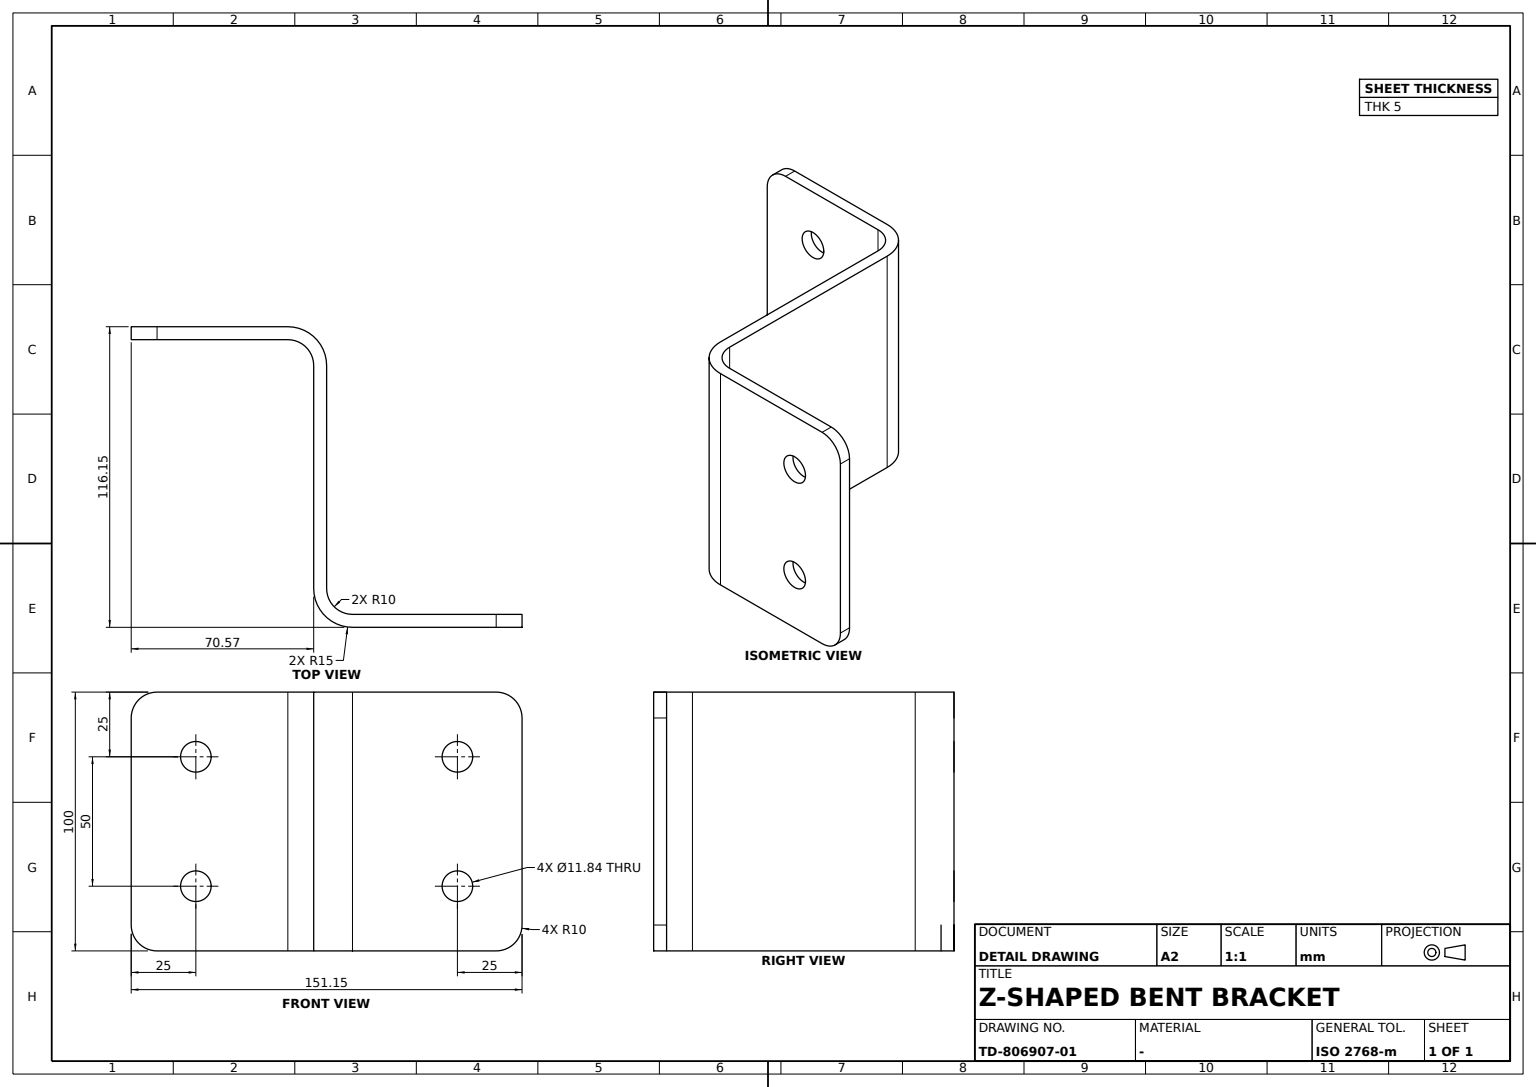
ISO-10303-21;
HEADER;
FILE_DESCRIPTION((''),'2;1');
FILE_NAME('','',(''),(''),'','','');
FILE_SCHEMA(('AUTOMOTIVE_DESIGN'));
ENDSEC;
DATA;
#1=APPLICATION_CONTEXT('');
#2=PRODUCT_CONTEXT('',#1,'mechanical');
#3=PRODUCT('','','',(#2));
#4=PRODUCT_DEFINITION_FORMATION('','',#3);
#5=PRODUCT_DEFINITION_CONTEXT('',#1,'design');
#6=PRODUCT_DEFINITION('','',#4,#5);
#7=PRODUCT_DEFINITION_SHAPE('','',#6);
#8=(LENGTH_UNIT()NAMED_UNIT(*)SI_UNIT(.MILLI.,.METRE.));
#9=(NAMED_UNIT(*)PLANE_ANGLE_UNIT()SI_UNIT($,.RADIAN.));
#10=(NAMED_UNIT(*)SI_UNIT($,.STERADIAN.)SOLID_ANGLE_UNIT());
#11=UNCERTAINTY_MEASURE_WITH_UNIT(LENGTH_MEASURE(0.005),#8,'distance_accuracy_value','');
#12=(GEOMETRIC_REPRESENTATION_CONTEXT(3)GLOBAL_UNCERTAINTY_ASSIGNED_CONTEXT((#11))GLOBAL_UNIT_ASSIGNED_CONTEXT((#8,#9,#10))REPRESENTATION_CONTEXT('',''));
#13=CARTESIAN_POINT('',(-175.5732,49.4268,40.));
#14=VERTEX_POINT('',#13);
#15=CARTESIAN_POINT('',(-175.5732,44.4268,40.));
#16=VERTEX_POINT('',#15);
#17=DIRECTION('',(0.,-1.,0.));
#18=VECTOR('',#17,1000.);
#19=LINE('',#13,#18);
#20=EDGE_CURVE('',#14,#16,#19,.T.);
#21=ORIENTED_EDGE('',*,*,#20,.F.);
#22=CARTESIAN_POINT('',(-175.5732,49.4268,-40.));
#23=VERTEX_POINT('',#22);
#24=CARTESIAN_POINT('',(-175.5732,49.4268,0.));
#25=DIRECTION('',(0.,0.,-1.));
#26=VECTOR('',#25,1000.);
#27=LINE('',#24,#26);
#28=EDGE_CURVE('',#14,#23,#27,.T.);
#29=ORIENTED_EDGE('',*,*,#28,.T.);
#30=CARTESIAN_POINT('',(-175.5732,44.4268,-40.));
#31=VERTEX_POINT('',#30);
#32=LINE('',#22,#18);
#33=EDGE_CURVE('',#23,#31,#32,.T.);
#34=ORIENTED_EDGE('',*,*,#33,.T.);
#35=CARTESIAN_POINT('',(-175.5732,44.4268,0.));
#36=LINE('',#35,#26);
#37=EDGE_CURVE('',#16,#31,#36,.T.);
#38=ORIENTED_EDGE('',*,*,#37,.F.);
#39=EDGE_LOOP('',(#21,#29,#34,#38));
#40=FACE_BOUND('',#39,.T.);
#41=CARTESIAN_POINT('',(-175.5732,49.4268,50.));
#42=DIRECTION('',(-1.,0.,0.));
#43=AXIS2_PLACEMENT_3D('',#41,#42,#25);
#44=PLANE('',#43);
#45=ADVANCED_FACE('',(#40),#44,.T.);
#46=CARTESIAN_POINT('',(-90.,-66.719599,50.));
#47=VERTEX_POINT('',#46);
#48=CARTESIAN_POINT('',(-90.,-66.719599,-50.));
#49=VERTEX_POINT('',#48);
#50=LINE('',#46,#26);
#51=EDGE_CURVE('',#47,#49,#50,.T.);
#52=ORIENTED_EDGE('',*,*,#51,.T.);
#53=CARTESIAN_POINT('',(-34.426804,-66.719599,-50.));
#54=VERTEX_POINT('',#53);
#55=CARTESIAN_POINT('',(-100.,-66.719599,-50.));
#56=DIRECTION('',(1.,0.,0.));
#57=VECTOR('',#56,1000.);
#58=LINE('',#55,#57);
#59=EDGE_CURVE('',#54,#49,#58,.F.);
#60=ORIENTED_EDGE('',*,*,#59,.F.);
#61=CARTESIAN_POINT('',(-24.4268,-66.719599,-40.));
#62=VERTEX_POINT('',#61);
#63=CARTESIAN_POINT('',(-34.4268,-66.719599,-40.));
#64=AXIS2_PLACEMENT_3D('',#63,#17,#56);
#65=CIRCLE('',#64,10.);
#66=EDGE_CURVE('',#62,#54,#65,.F.);
#67=ORIENTED_EDGE('',*,*,#66,.F.);
#68=CARTESIAN_POINT('',(-24.4268,-66.719599,40.));
#69=VERTEX_POINT('',#68);
#70=CARTESIAN_POINT('',(-24.4268,-66.719599,0.));
#71=DIRECTION('',(0.,0.,1.));
#72=VECTOR('',#71,1000.);
#73=LINE('',#70,#72);
#74=EDGE_CURVE('',#62,#69,#73,.T.);
#75=ORIENTED_EDGE('',*,*,#74,.T.);
#76=CARTESIAN_POINT('',(-34.4268,-66.719599,50.));
#77=VERTEX_POINT('',#76);
#78=CARTESIAN_POINT('',(-34.4268,-66.719599,40.));
#79=AXIS2_PLACEMENT_3D('',#78,#17,#56);
#80=CIRCLE('',#79,10.);
#81=EDGE_CURVE('',#77,#69,#80,.F.);
#82=ORIENTED_EDGE('',*,*,#81,.F.);
#83=CARTESIAN_POINT('',(0.,-66.719599,50.));
#84=LINE('',#83,#57);
#85=EDGE_CURVE('',#47,#77,#84,.T.);
#86=ORIENTED_EDGE('',*,*,#85,.F.);
#87=EDGE_LOOP('',(#52,#60,#67,#75,#82,#86));
#88=FACE_BOUND('',#87,.T.);
#89=CARTESIAN_POINT('',(-43.5093,-66.719599,25.));
#90=VERTEX_POINT('',#89);
#91=CARTESIAN_POINT('',(-49.4268,-66.719599,25.));
#92=AXIS2_PLACEMENT_3D('',#91,#17,#56);
#93=CIRCLE('',#92,5.9175);
#94=EDGE_CURVE('',#90,#90,#93,.T.);
#95=ORIENTED_EDGE('',*,*,#94,.F.);
#96=EDGE_LOOP('',(#95));
#97=FACE_BOUND('',#96,.T.);
#98=CARTESIAN_POINT('',(-43.5093,-66.719599,-25.));
#99=VERTEX_POINT('',#98);
#100=CARTESIAN_POINT('',(-49.4268,-66.719599,-25.));
#101=AXIS2_PLACEMENT_3D('',#100,#17,#56);
#102=CIRCLE('',#101,5.9175);
#103=EDGE_CURVE('',#99,#99,#102,.T.);
#104=ORIENTED_EDGE('',*,*,#103,.F.);
#105=EDGE_LOOP('',(#104));
#106=FACE_BOUND('',#105,.T.);
#107=CARTESIAN_POINT('',(-149.4268,-66.719599,0.));
#108=AXIS2_PLACEMENT_3D('',#107,#17,#56);
#109=PLANE('',#108);
#110=ADVANCED_FACE('',(#88,#97,#106),#109,.T.);
#111=CARTESIAN_POINT('',(-24.4268,-61.719599,-40.));
#112=VERTEX_POINT('',#111);
#113=LINE('',#111,#18);
#114=EDGE_CURVE('',#112,#62,#113,.T.);
#115=ORIENTED_EDGE('',*,*,#114,.F.);
#116=CARTESIAN_POINT('',(-24.4268,-61.719599,40.));
#117=VERTEX_POINT('',#116);
#118=CARTESIAN_POINT('',(-24.4268,-61.719599,0.));
#119=LINE('',#118,#72);
#120=EDGE_CURVE('',#112,#117,#119,.T.);
#121=ORIENTED_EDGE('',*,*,#120,.T.);
#122=LINE('',#116,#18);
#123=EDGE_CURVE('',#117,#69,#122,.T.);
#124=ORIENTED_EDGE('',*,*,#123,.T.);
#125=ORIENTED_EDGE('',*,*,#74,.F.);
#126=EDGE_LOOP('',(#115,#121,#124,#125));
#127=FACE_BOUND('',#126,.T.);
#128=CARTESIAN_POINT('',(-24.4268,-61.719599,-50.));
#129=AXIS2_PLACEMENT_3D('',#128,#56,#71);
#130=PLANE('',#129);
#131=ADVANCED_FACE('',(#127),#130,.T.);
#132=CARTESIAN_POINT('',(-105.,34.4268,50.));
#133=VERTEX_POINT('',#132);
#134=CARTESIAN_POINT('',(-105.,34.4268,-50.));
#135=VERTEX_POINT('',#134);
#136=LINE('',#132,#26);
#137=EDGE_CURVE('',#133,#135,#136,.T.);
#138=ORIENTED_EDGE('',*,*,#137,.T.);
#139=CARTESIAN_POINT('',(-105.,-51.719599,-50.));
#140=VERTEX_POINT('',#139);
#141=LINE('',#134,#18);
#142=EDGE_CURVE('',#140,#135,#141,.F.);
#143=ORIENTED_EDGE('',*,*,#142,.F.);
#144=CARTESIAN_POINT('',(-105.,-51.719599,50.));
#145=VERTEX_POINT('',#144);
#146=LINE('',#144,#26);
#147=EDGE_CURVE('',#145,#140,#146,.T.);
#148=ORIENTED_EDGE('',*,*,#147,.F.);
#149=CARTESIAN_POINT('',(-105.,125.,50.));
#150=LINE('',#149,#18);
#151=EDGE_CURVE('',#133,#145,#150,.T.);
#152=ORIENTED_EDGE('',*,*,#151,.F.);
#153=EDGE_LOOP('',(#138,#143,#148,#152));
#154=FACE_BOUND('',#153,.T.);
#155=CARTESIAN_POINT('',(-105.,-11.146399,0.));
#156=AXIS2_PLACEMENT_3D('',#155,#42,#17);
#157=PLANE('',#156);
#158=ADVANCED_FACE('',(#154),#157,.T.);
#159=CARTESIAN_POINT('',(-144.6557,49.4268,25.));
#160=VERTEX_POINT('',#159);
#161=CARTESIAN_POINT('',(-150.5732,49.4268,25.));
#162=AXIS2_PLACEMENT_3D('',#161,#17,#56);
#163=CIRCLE('',#162,5.9175);
#164=EDGE_CURVE('',#160,#160,#163,.T.);
#165=ORIENTED_EDGE('',*,*,#164,.F.);
#166=EDGE_LOOP('',(#165));
#167=FACE_BOUND('',#166,.T.);
#168=CARTESIAN_POINT('',(-144.6557,44.4268,25.));
#169=VERTEX_POINT('',#168);
#170=CARTESIAN_POINT('',(-150.5732,44.4268,25.));
#171=AXIS2_PLACEMENT_3D('',#170,#17,#56);
#172=CIRCLE('',#171,5.9175);
#173=EDGE_CURVE('',#169,#169,#172,.T.);
#174=ORIENTED_EDGE('',*,*,#173,.T.);
#175=EDGE_LOOP('',(#174));
#176=FACE_BOUND('',#175,.T.);
#177=CARTESIAN_POINT('',(-150.5732,46.9268,25.));
#178=AXIS2_PLACEMENT_3D('',#177,#17,#56);
#179=CYLINDRICAL_SURFACE('',#178,5.9175);
#180=ADVANCED_FACE('',(#167,#176),#179,.F.);
#181=CARTESIAN_POINT('',(-100.,-51.719599,50.));
#182=VERTEX_POINT('',#181);
#183=CARTESIAN_POINT('',(-100.,-51.719599,-50.));
#184=VERTEX_POINT('',#183);
#185=LINE('',#181,#26);
#186=EDGE_CURVE('',#182,#184,#185,.T.);
#187=ORIENTED_EDGE('',*,*,#186,.T.);
#188=CARTESIAN_POINT('',(-100.,34.4268,-50.));
#189=VERTEX_POINT('',#188);
#190=LINE('',#188,#18);
#191=EDGE_CURVE('',#184,#189,#190,.F.);
#192=ORIENTED_EDGE('',*,*,#191,.T.);
#193=CARTESIAN_POINT('',(-100.,34.4268,50.));
#194=VERTEX_POINT('',#193);
#195=LINE('',#193,#26);
#196=EDGE_CURVE('',#194,#189,#195,.T.);
#197=ORIENTED_EDGE('',*,*,#196,.F.);
#198=CARTESIAN_POINT('',(-100.,125.,50.));
#199=LINE('',#198,#18);
#200=EDGE_CURVE('',#194,#182,#199,.T.);
#201=ORIENTED_EDGE('',*,*,#200,.T.);
#202=EDGE_LOOP('',(#187,#192,#197,#201));
#203=FACE_BOUND('',#202,.T.);
#204=CARTESIAN_POINT('',(-100.,-11.146399,0.));
#205=AXIS2_PLACEMENT_3D('',#204,#42,#17);
#206=PLANE('',#205);
#207=ADVANCED_FACE('',(#203),#206,.F.);
#208=CARTESIAN_POINT('',(-34.4268,-61.719599,-50.));
#209=VERTEX_POINT('',#208);
#210=LINE('',#208,#18);
#211=EDGE_CURVE('',#209,#54,#210,.T.);
#212=ORIENTED_EDGE('',*,*,#211,.F.);
#213=CARTESIAN_POINT('',(-34.4268,-61.719599,-40.));
#214=AXIS2_PLACEMENT_3D('',#213,#17,#56);
#215=CIRCLE('',#214,10.);
#216=EDGE_CURVE('',#112,#209,#215,.F.);
#217=ORIENTED_EDGE('',*,*,#216,.F.);
#218=ORIENTED_EDGE('',*,*,#114,.T.);
#219=ORIENTED_EDGE('',*,*,#66,.T.);
#220=EDGE_LOOP('',(#212,#217,#218,#219));
#221=FACE_BOUND('',#220,.T.);
#222=CYLINDRICAL_SURFACE('',#214,10.);
#223=ADVANCED_FACE('',(#221),#222,.T.);
#224=CARTESIAN_POINT('',(-165.5732,44.4268,50.));
#225=VERTEX_POINT('',#224);
#226=CARTESIAN_POINT('',(-165.5732,44.4268,40.));
#227=AXIS2_PLACEMENT_3D('',#226,#17,#56);
#228=CIRCLE('',#227,10.);
#229=EDGE_CURVE('',#16,#225,#228,.F.);
#230=ORIENTED_EDGE('',*,*,#229,.T.);
#231=CARTESIAN_POINT('',(-165.5732,49.4268,50.));
#232=VERTEX_POINT('',#231);
#233=LINE('',#231,#18);
#234=EDGE_CURVE('',#232,#225,#233,.T.);
#235=ORIENTED_EDGE('',*,*,#234,.F.);
#236=CARTESIAN_POINT('',(-165.5732,49.4268,40.));
#237=AXIS2_PLACEMENT_3D('',#236,#17,#56);
#238=CIRCLE('',#237,10.);
#239=EDGE_CURVE('',#14,#232,#238,.F.);
#240=ORIENTED_EDGE('',*,*,#239,.F.);
#241=ORIENTED_EDGE('',*,*,#20,.T.);
#242=EDGE_LOOP('',(#230,#235,#240,#241));
#243=FACE_BOUND('',#242,.T.);
#244=CYLINDRICAL_SURFACE('',#237,10.);
#245=ADVANCED_FACE('',(#243),#244,.T.);
#246=CARTESIAN_POINT('',(-43.5093,-61.719599,-25.));
#247=VERTEX_POINT('',#246);
#248=CARTESIAN_POINT('',(-49.4268,-61.719599,-25.));
#249=AXIS2_PLACEMENT_3D('',#248,#17,#56);
#250=CIRCLE('',#249,5.9175);
#251=EDGE_CURVE('',#247,#247,#250,.T.);
#252=ORIENTED_EDGE('',*,*,#251,.T.);
#253=EDGE_LOOP('',(#252));
#254=FACE_BOUND('',#253,.T.);
#255=CARTESIAN_POINT('',(-90.,-61.719599,-50.));
#256=VERTEX_POINT('',#255);
#257=CARTESIAN_POINT('',(-100.,-61.719599,-50.));
#258=LINE('',#257,#57);
#259=EDGE_CURVE('',#209,#256,#258,.F.);
#260=ORIENTED_EDGE('',*,*,#259,.T.);
#261=CARTESIAN_POINT('',(-90.,-61.719599,50.));
#262=VERTEX_POINT('',#261);
#263=LINE('',#261,#26);
#264=EDGE_CURVE('',#262,#256,#263,.T.);
#265=ORIENTED_EDGE('',*,*,#264,.F.);
#266=CARTESIAN_POINT('',(-34.4268,-61.719599,50.));
#267=VERTEX_POINT('',#266);
#268=CARTESIAN_POINT('',(0.,-61.719599,50.));
#269=LINE('',#268,#57);
#270=EDGE_CURVE('',#262,#267,#269,.T.);
#271=ORIENTED_EDGE('',*,*,#270,.T.);
#272=CARTESIAN_POINT('',(-34.4268,-61.719599,40.));
#273=AXIS2_PLACEMENT_3D('',#272,#17,#56);
#274=CIRCLE('',#273,10.);
#275=EDGE_CURVE('',#267,#117,#274,.F.);
#276=ORIENTED_EDGE('',*,*,#275,.T.);
#277=ORIENTED_EDGE('',*,*,#120,.F.);
#278=ORIENTED_EDGE('',*,*,#216,.T.);
#279=EDGE_LOOP('',(#260,#265,#271,#276,#277,#278));
#280=FACE_BOUND('',#279,.T.);
#281=CARTESIAN_POINT('',(-43.5093,-61.719599,25.));
#282=VERTEX_POINT('',#281);
#283=CARTESIAN_POINT('',(-49.4268,-61.719599,25.));
#284=AXIS2_PLACEMENT_3D('',#283,#17,#56);
#285=CIRCLE('',#284,5.9175);
#286=EDGE_CURVE('',#282,#282,#285,.T.);
#287=ORIENTED_EDGE('',*,*,#286,.T.);
#288=EDGE_LOOP('',(#287));
#289=FACE_BOUND('',#288,.T.);
#290=CARTESIAN_POINT('',(-149.4268,-61.719599,0.));
#291=AXIS2_PLACEMENT_3D('',#290,#17,#56);
#292=PLANE('',#291);
#293=ADVANCED_FACE('',(#254,#280,#289),#292,.F.);
#294=ORIENTED_EDGE('',*,*,#239,.T.);
#295=CARTESIAN_POINT('',(-115.,49.4268,50.));
#296=VERTEX_POINT('',#295);
#297=CARTESIAN_POINT('',(0.,49.4268,50.));
#298=LINE('',#297,#57);
#299=EDGE_CURVE('',#232,#296,#298,.T.);
#300=ORIENTED_EDGE('',*,*,#299,.T.);
#301=CARTESIAN_POINT('',(-115.,49.4268,-50.));
#302=VERTEX_POINT('',#301);
#303=LINE('',#295,#26);
#304=EDGE_CURVE('',#296,#302,#303,.T.);
#305=ORIENTED_EDGE('',*,*,#304,.T.);
#306=CARTESIAN_POINT('',(-165.573196,49.4268,-50.));
#307=VERTEX_POINT('',#306);
#308=CARTESIAN_POINT('',(-100.,49.4268,-50.));
#309=LINE('',#308,#57);
#310=EDGE_CURVE('',#302,#307,#309,.F.);
#311=ORIENTED_EDGE('',*,*,#310,.T.);
#312=CARTESIAN_POINT('',(-165.5732,49.4268,-40.));
#313=AXIS2_PLACEMENT_3D('',#312,#17,#56);
#314=CIRCLE('',#313,10.);
#315=EDGE_CURVE('',#307,#23,#314,.F.);
#316=ORIENTED_EDGE('',*,*,#315,.T.);
#317=ORIENTED_EDGE('',*,*,#28,.F.);
#318=EDGE_LOOP('',(#294,#300,#305,#311,#316,#317));
#319=FACE_BOUND('',#318,.T.);
#320=CARTESIAN_POINT('',(-144.6557,49.4268,-25.));
#321=VERTEX_POINT('',#320);
#322=CARTESIAN_POINT('',(-150.5732,49.4268,-25.));
#323=AXIS2_PLACEMENT_3D('',#322,#17,#56);
#324=CIRCLE('',#323,5.9175);
#325=EDGE_CURVE('',#321,#321,#324,.T.);
#326=ORIENTED_EDGE('',*,*,#325,.T.);
#327=EDGE_LOOP('',(#326));
#328=FACE_BOUND('',#327,.T.);
#329=ORIENTED_EDGE('',*,*,#164,.T.);
#330=EDGE_LOOP('',(#329));
#331=FACE_BOUND('',#330,.T.);
#332=CARTESIAN_POINT('',(-50.5732,49.4268,0.));
#333=AXIS2_PLACEMENT_3D('',#332,#17,#56);
#334=PLANE('',#333);
#335=ADVANCED_FACE('',(#319,#328,#331),#334,.F.);
#336=ORIENTED_EDGE('',*,*,#173,.F.);
#337=EDGE_LOOP('',(#336));
#338=FACE_BOUND('',#337,.T.);
#339=CARTESIAN_POINT('',(-144.6557,44.4268,-25.));
#340=VERTEX_POINT('',#339);
#341=CARTESIAN_POINT('',(-150.5732,44.4268,-25.));
#342=AXIS2_PLACEMENT_3D('',#341,#17,#56);
#343=CIRCLE('',#342,5.9175);
#344=EDGE_CURVE('',#340,#340,#343,.T.);
#345=ORIENTED_EDGE('',*,*,#344,.F.);
#346=EDGE_LOOP('',(#345));
#347=FACE_BOUND('',#346,.T.);
#348=ORIENTED_EDGE('',*,*,#229,.F.);
#349=ORIENTED_EDGE('',*,*,#37,.T.);
#350=CARTESIAN_POINT('',(-165.5732,44.4268,-50.));
#351=VERTEX_POINT('',#350);
#352=CARTESIAN_POINT('',(-165.5732,44.4268,-40.));
#353=AXIS2_PLACEMENT_3D('',#352,#17,#56);
#354=CIRCLE('',#353,10.);
#355=EDGE_CURVE('',#351,#31,#354,.F.);
#356=ORIENTED_EDGE('',*,*,#355,.F.);
#357=CARTESIAN_POINT('',(-115.,44.4268,-50.));
#358=VERTEX_POINT('',#357);
#359=CARTESIAN_POINT('',(-100.,44.4268,-50.));
#360=LINE('',#359,#57);
#361=EDGE_CURVE('',#358,#351,#360,.F.);
#362=ORIENTED_EDGE('',*,*,#361,.F.);
#363=CARTESIAN_POINT('',(-115.,44.4268,50.));
#364=VERTEX_POINT('',#363);
#365=LINE('',#363,#26);
#366=EDGE_CURVE('',#364,#358,#365,.T.);
#367=ORIENTED_EDGE('',*,*,#366,.F.);
#368=CARTESIAN_POINT('',(0.,44.4268,50.));
#369=LINE('',#368,#57);
#370=EDGE_CURVE('',#225,#364,#369,.T.);
#371=ORIENTED_EDGE('',*,*,#370,.F.);
#372=EDGE_LOOP('',(#348,#349,#356,#362,#367,#371));
#373=FACE_BOUND('',#372,.T.);
#374=CARTESIAN_POINT('',(-50.5732,44.4268,0.));
#375=AXIS2_PLACEMENT_3D('',#374,#17,#56);
#376=PLANE('',#375);
#377=ADVANCED_FACE('',(#338,#347,#373),#376,.T.);
#378=CARTESIAN_POINT('',(-115.,34.4268,50.));
#379=AXIS2_PLACEMENT_3D('',#378,#71,#56);
#380=CIRCLE('',#379,15.);
#381=EDGE_CURVE('',#194,#296,#380,.T.);
#382=ORIENTED_EDGE('',*,*,#381,.F.);
#383=ORIENTED_EDGE('',*,*,#196,.T.);
#384=CARTESIAN_POINT('',(-115.,34.4268,-50.));
#385=AXIS2_PLACEMENT_3D('',#384,#71,#56);
#386=CIRCLE('',#385,15.);
#387=EDGE_CURVE('',#189,#302,#386,.T.);
#388=ORIENTED_EDGE('',*,*,#387,.T.);
#389=ORIENTED_EDGE('',*,*,#304,.F.);
#390=EDGE_LOOP('',(#382,#383,#388,#389));
#391=FACE_BOUND('',#390,.T.);
#392=DIRECTION('',(0.,1.,0.));
#393=AXIS2_PLACEMENT_3D('',#378,#25,#392);
#394=CYLINDRICAL_SURFACE('',#393,15.);
#395=ADVANCED_FACE('',(#391),#394,.T.);
#396=CARTESIAN_POINT('',(-90.,-51.719599,-50.));
#397=AXIS2_PLACEMENT_3D('',#396,#71,#56);
#398=CIRCLE('',#397,10.);
#399=EDGE_CURVE('',#184,#256,#398,.T.);
#400=ORIENTED_EDGE('',*,*,#399,.T.);
#401=ORIENTED_EDGE('',*,*,#259,.F.);
#402=ORIENTED_EDGE('',*,*,#211,.T.);
#403=ORIENTED_EDGE('',*,*,#59,.T.);
#404=CIRCLE('',#397,15.);
#405=EDGE_CURVE('',#140,#49,#404,.T.);
#406=ORIENTED_EDGE('',*,*,#405,.F.);
#407=ORIENTED_EDGE('',*,*,#142,.T.);
#408=CIRCLE('',#385,10.);
#409=EDGE_CURVE('',#135,#358,#408,.T.);
#410=ORIENTED_EDGE('',*,*,#409,.T.);
#411=ORIENTED_EDGE('',*,*,#361,.T.);
#412=CARTESIAN_POINT('',(-165.5732,49.4268,-50.));
#413=LINE('',#412,#18);
#414=EDGE_CURVE('',#307,#351,#413,.T.);
#415=ORIENTED_EDGE('',*,*,#414,.F.);
#416=ORIENTED_EDGE('',*,*,#310,.F.);
#417=ORIENTED_EDGE('',*,*,#387,.F.);
#418=ORIENTED_EDGE('',*,*,#191,.F.);
#419=EDGE_LOOP('',(#400,#401,#402,#403,#406,#407,#410,#411,#415,#416,#417,#418));
#420=FACE_BOUND('',#419,.T.);
#421=DIRECTION('',(-0.382683432,0.923879533,0.));
#422=AXIS2_PLACEMENT_3D('',#188,#71,#421);
#423=PLANE('',#422);
#424=ADVANCED_FACE('',(#420),#423,.F.);
#425=LINE('',#266,#18);
#426=EDGE_CURVE('',#267,#77,#425,.T.);
#427=ORIENTED_EDGE('',*,*,#426,.T.);
#428=ORIENTED_EDGE('',*,*,#81,.T.);
#429=ORIENTED_EDGE('',*,*,#123,.F.);
#430=ORIENTED_EDGE('',*,*,#275,.F.);
#431=EDGE_LOOP('',(#427,#428,#429,#430));
#432=FACE_BOUND('',#431,.T.);
#433=CYLINDRICAL_SURFACE('',#273,10.);
#434=ADVANCED_FACE('',(#432),#433,.T.);
#435=ORIENTED_EDGE('',*,*,#33,.F.);
#436=ORIENTED_EDGE('',*,*,#315,.F.);
#437=ORIENTED_EDGE('',*,*,#414,.T.);
#438=ORIENTED_EDGE('',*,*,#355,.T.);
#439=EDGE_LOOP('',(#435,#436,#437,#438));
#440=FACE_BOUND('',#439,.T.);
#441=CYLINDRICAL_SURFACE('',#313,10.);
#442=ADVANCED_FACE('',(#440),#441,.T.);
#443=ORIENTED_EDGE('',*,*,#137,.F.);
#444=CIRCLE('',#379,10.);
#445=EDGE_CURVE('',#133,#364,#444,.T.);
#446=ORIENTED_EDGE('',*,*,#445,.T.);
#447=ORIENTED_EDGE('',*,*,#366,.T.);
#448=ORIENTED_EDGE('',*,*,#409,.F.);
#449=EDGE_LOOP('',(#443,#446,#447,#448));
#450=FACE_BOUND('',#449,.T.);
#451=CYLINDRICAL_SURFACE('',#393,10.);
#452=ADVANCED_FACE('',(#450),#451,.F.);
#453=ORIENTED_EDGE('',*,*,#85,.T.);
#454=ORIENTED_EDGE('',*,*,#426,.F.);
#455=ORIENTED_EDGE('',*,*,#270,.F.);
#456=CARTESIAN_POINT('',(-90.,-51.719599,50.));
#457=AXIS2_PLACEMENT_3D('',#456,#71,#56);
#458=CIRCLE('',#457,10.);
#459=EDGE_CURVE('',#182,#262,#458,.T.);
#460=ORIENTED_EDGE('',*,*,#459,.F.);
#461=ORIENTED_EDGE('',*,*,#200,.F.);
#462=ORIENTED_EDGE('',*,*,#381,.T.);
#463=ORIENTED_EDGE('',*,*,#299,.F.);
#464=ORIENTED_EDGE('',*,*,#234,.T.);
#465=ORIENTED_EDGE('',*,*,#370,.T.);
#466=ORIENTED_EDGE('',*,*,#445,.F.);
#467=ORIENTED_EDGE('',*,*,#151,.T.);
#468=CIRCLE('',#457,15.);
#469=EDGE_CURVE('',#145,#47,#468,.T.);
#470=ORIENTED_EDGE('',*,*,#469,.T.);
#471=EDGE_LOOP('',(#453,#454,#455,#460,#461,#462,#463,#464,#465,#466,#467,#470));
#472=FACE_BOUND('',#471,.T.);
#473=CARTESIAN_POINT('',(0.,125.,50.));
#474=AXIS2_PLACEMENT_3D('',#473,#71,#17);
#475=PLANE('',#474);
#476=ADVANCED_FACE('',(#472),#475,.T.);
#477=ORIENTED_EDGE('',*,*,#344,.T.);
#478=EDGE_LOOP('',(#477));
#479=FACE_BOUND('',#478,.T.);
#480=ORIENTED_EDGE('',*,*,#325,.F.);
#481=EDGE_LOOP('',(#480));
#482=FACE_BOUND('',#481,.T.);
#483=CARTESIAN_POINT('',(-150.5732,46.9268,-25.));
#484=AXIS2_PLACEMENT_3D('',#483,#17,#56);
#485=CYLINDRICAL_SURFACE('',#484,5.9175);
#486=ADVANCED_FACE('',(#479,#482),#485,.F.);
#487=ORIENTED_EDGE('',*,*,#286,.F.);
#488=EDGE_LOOP('',(#487));
#489=FACE_BOUND('',#488,.T.);
#490=ORIENTED_EDGE('',*,*,#94,.T.);
#491=EDGE_LOOP('',(#490));
#492=FACE_BOUND('',#491,.T.);
#493=CARTESIAN_POINT('',(-49.4268,-64.219599,25.));
#494=AXIS2_PLACEMENT_3D('',#493,#17,#56);
#495=CYLINDRICAL_SURFACE('',#494,5.9175);
#496=ADVANCED_FACE('',(#489,#492),#495,.F.);
#497=ORIENTED_EDGE('',*,*,#147,.T.);
#498=ORIENTED_EDGE('',*,*,#405,.T.);
#499=ORIENTED_EDGE('',*,*,#51,.F.);
#500=ORIENTED_EDGE('',*,*,#469,.F.);
#501=EDGE_LOOP('',(#497,#498,#499,#500));
#502=FACE_BOUND('',#501,.T.);
#503=AXIS2_PLACEMENT_3D('',#456,#25,#17);
#504=CYLINDRICAL_SURFACE('',#503,15.);
#505=ADVANCED_FACE('',(#502),#504,.T.);
#506=ORIENTED_EDGE('',*,*,#103,.T.);
#507=EDGE_LOOP('',(#506));
#508=FACE_BOUND('',#507,.T.);
#509=ORIENTED_EDGE('',*,*,#251,.F.);
#510=EDGE_LOOP('',(#509));
#511=FACE_BOUND('',#510,.T.);
#512=CARTESIAN_POINT('',(-49.4268,-64.219599,-25.));
#513=AXIS2_PLACEMENT_3D('',#512,#17,#56);
#514=CYLINDRICAL_SURFACE('',#513,5.9175);
#515=ADVANCED_FACE('',(#508,#511),#514,.F.);
#516=ORIENTED_EDGE('',*,*,#186,.F.);
#517=ORIENTED_EDGE('',*,*,#459,.T.);
#518=ORIENTED_EDGE('',*,*,#264,.T.);
#519=ORIENTED_EDGE('',*,*,#399,.F.);
#520=EDGE_LOOP('',(#516,#517,#518,#519));
#521=FACE_BOUND('',#520,.T.);
#522=CYLINDRICAL_SURFACE('',#503,10.);
#523=ADVANCED_FACE('',(#521),#522,.F.);
#524=CLOSED_SHELL('',(#45,#110,#131,#158,#180,#207,#223,#245,#293,#335,#377,#395,#424,#434,#442,#452,#476,#486,#496,#505,#515,#523));
#525=MANIFOLD_SOLID_BREP('',#524);
#526=ADVANCED_BREP_SHAPE_REPRESENTATION('',(#525),#12);
#527=SHAPE_DEFINITION_REPRESENTATION(#7,#526);
ENDSEC;
END-ISO-10303-21;
